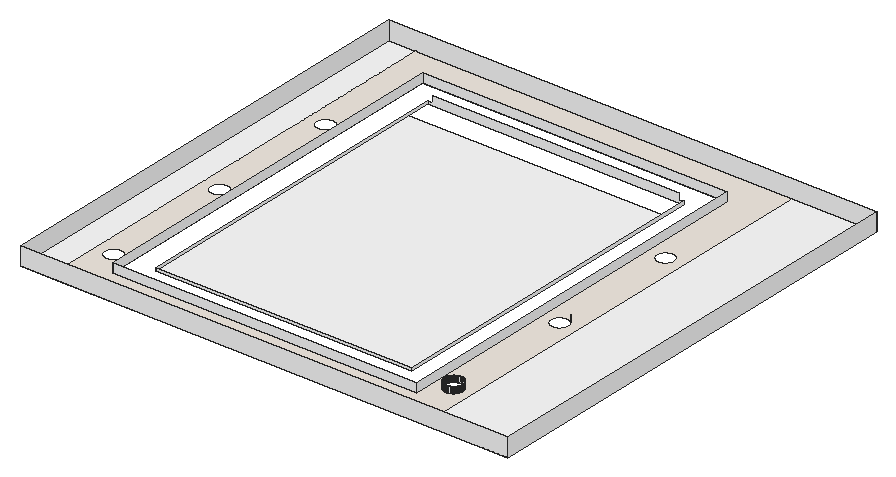
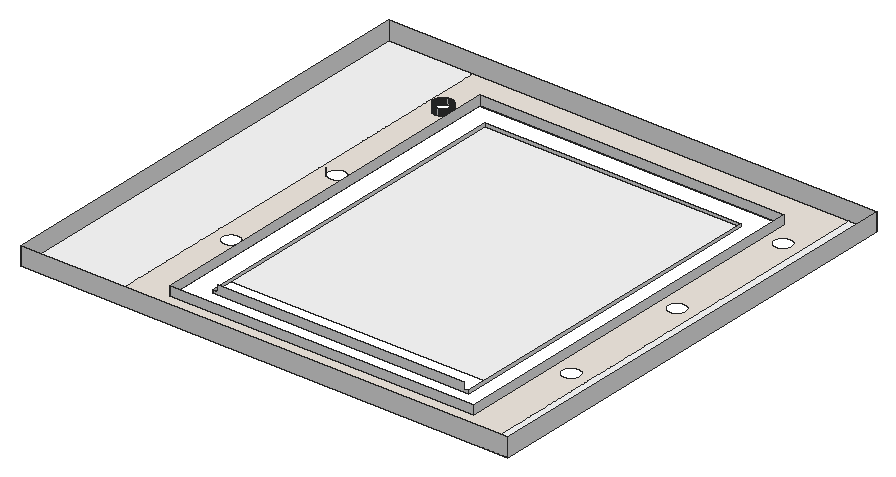
# SketchUp Ruby script. Lengths in inches.
U = 1.inch
M = Sketchup.active_model
def pt(a) = Geom::Point3d.new(a.map { |v| v * U })
def face(e, loops, mat)
  f = e.add_face(loops[0].map { |a| pt(a) })
  loops[1..].each { |l| e.add_face(l.map { |a| pt(a) }).erase! }
  f.material = f.back_material = mat if mat
  f
end
# faces: each face lists its corners as indices into pts; further lists are holes
def faces(e, pts, list, mat = nil) = list.each { |f| face(e, (f[0].is_a?(Array) ? f : [f]).map { |l| l.map { |i| pts[i] } }, mat) }
# xy, xz, yz: faces in a plane at the given z, y or x. An outline is a flat list of corners, or four numbers for a rectangle; further outlines are holes
def ring(l) = l.size == 4 ? [[l[0], l[1]], [l[2], l[1]], [l[2], l[3]], [l[0], l[3]]] : l.each_slice(2).to_a
def flat(e, list, mat, &to3) = list.each { |f| face(e, (f[0].is_a?(Array) ? f : [f]).map { |l| ring(l).map { |u, v| to3.(u, v) } }, mat) }
def xy(e, z, list, mat = nil) = flat(e, list, mat) { |x, y| [x, y, z] }
def xz(e, y, list, mat = nil) = flat(e, list, mat) { |x, z| [x, y, z] }
def yz(e, x, list, mat = nil) = flat(e, list, mat) { |y, z| [x, y, z] }
def lines(e, pts, list) = list.each { |a, b| e.add_line(pt(pts[a]), pt(pts[b])) }
# prism: a flat outline (further loops are holes) pulled along v
def prism(e, loops, v, mat = nil)
  f = face(e, loops, mat); d = Geom::Vector3d.new(v.map { |x| x * U })
  f.pushpull(f.normal.samedirection?(d) ? d.length : -d.length)
end
def box(e, o, s, mat = nil) = prism(e, [[o, [o[0] + s[0], o[1], o[2]], [o[0] + s[0], o[1] + s[1], o[2]], [o[0], o[1] + s[1], o[2]]]], [0, 0, s[2]], mat)
def at(x, y, z, deg = 0) = Geom::Transformation.translation(pt([x, y, z])) * Geom::Transformation.rotation(ORIGIN, Z_AXIS, deg.degrees)
def axes(o, x, y, z) = Geom::Transformation.new([*x, 0, *y, 0, *z, 0, *pt(o).to_a, 1])
def part(name) = M.definitions.add(name)
# library, detail: a bought-in or finely detailed component or shape, given as its bounding box
def library(name, o, s) = part(name).tap { |d| box(d.entities, o, s) }
def detail(e, o, s) = box(e.add_group.entities, o, s)
def put(e, d, t, mat = nil) = e.add_instance(d, t).tap { |i| i.material = mat if mat }
def group(e, t, mat = nil) = e.add_group.tap { |g| g.transformation = t; g.material = mat if mat }.entities
root = M.entities
M.materials.add("[Color M00]").color = [255, 255, 255]
M.materials.add("[Formica Laminate Light]").color = [242, 234, 226]
xy(root,120,[[0,0,9,153],[134,0,162,153],[29,20,114,125]],"[Color M00]")
xy(root,120,[[[9,0,134,153],[21,12,122,141],[14.87,105,15.0625,105,15.25,105.01,15.4375,105.03,15.62,105.07,15.81,105.11,15.98,105.17,16.16,105.23,16.33,105.3125,16.5,105.4,16.66,105.5,16.8125,105.61,16.96,105.73,17.1,105.86,17.23,105.99,17.35,106.14,17.57,106.44,17.66,106.61,17.74,106.78,17.8125,106.95,17.87,107.13,17.92,107.3125,17.96,107.5,17.98,107.68,18,107.87,18,108.0625,17.99,108.25,17.97,108.4375,17.93,108.62,17.89,108.81,17.83,108.98,17.77,109.16,17.6875,109.33,17.6,109.5,17.5,109.66,17.39,109.8125,17.27,109.96,17.14,110.1,17.01,110.23,16.86,110.35,16.56,110.57,16.39,110.66,16.22,110.74,16.05,110.8125,15.87,110.87,15.6875,110.92,15.5,110.96,15.32,110.98,15.13,111,14.9375,111,14.75,110.99,14.5625,110.97,14.38,110.93,14.19,110.89,14.02,110.83,13.84,110.77,13.67,110.6875,13.5,110.6,13.34,110.5,13.1875,110.39,13.04,110.27,12.9,110.14,12.77,110.01,12.65,109.86,12.43,109.56,12.34,109.39,12.26,109.22,12.1875,109.05,12.13,108.87,12.08,108.6875,12.04,108.5,12.02,108.32,12,108.13,12,107.9375,12.01,107.75,12.03,107.5625,12.07,107.38,12.11,107.19,12.17,107.02,12.23,106.84,12.3125,106.67,12.4,106.5,12.5,106.34,12.61,106.1875,12.73,106.04,12.86,105.9,12.99,105.77,13.14,105.65,13.44,105.43,13.61,105.34,13.78,105.26,13.95,105.1875,14.13,105.13,14.3125,105.08,14.5,105.04,14.68,105.02],[14.87,17,15.0625,17,15.25,17.01,15.4375,17.03,15.62,17.07,15.81,17.11,15.98,17.17,16.16,17.23,16.33,17.3125,16.5,17.4,16.66,17.5,16.8125,17.61,16.96,17.73,17.1,17.86,17.23,17.99,17.35,18.14,17.57,18.44,17.66,18.61,17.74,18.78,17.8125,18.95,17.87,19.13,17.92,19.3125,17.96,19.5,17.98,19.68,18,19.87,18,20.0625,17.99,20.25,17.97,20.4375,17.93,20.62,17.89,20.81,17.83,20.98,17.77,21.16,17.6875,21.33,17.6,21.5,17.5,21.66,17.39,21.8125,17.27,21.96,17.14,22.1,17.01,22.23,16.86,22.35,16.56,22.57,16.39,22.66,16.22,22.74,16.05,22.8125,15.87,22.87,15.6875,22.92,15.5,22.96,15.32,22.98,15.13,23,14.9375,23,14.75,22.99,14.5625,22.97,14.38,22.93,14.19,22.89,14.02,22.83,13.84,22.77,13.67,22.6875,13.5,22.6,13.34,22.5,13.1875,22.39,13.04,22.27,12.9,22.14,12.77,22.01,12.65,21.86,12.43,21.56,12.34,21.39,12.26,21.22,12.1875,21.05,12.13,20.87,12.08,20.6875,12.04,20.5,12.02,20.32,12,20.13,12,19.9375,12.01,19.75,12.03,19.5625,12.07,19.38,12.11,19.19,12.17,19.02,12.23,18.84,12.3125,18.67,12.4,18.5,12.5,18.34,12.61,18.1875,12.73,18.04,12.86,17.9,12.99,17.77,13.14,17.65,13.44,17.43,13.61,17.34,13.78,17.26,13.95,17.1875,14.13,17.13,14.3125,17.08,14.5,17.04,14.68,17.02],[14.87,61,15.0625,61,15.25,61.01,15.4375,61.03,15.62,61.07,15.81,61.11,15.98,61.17,16.16,61.23,16.33,61.3125,16.5,61.4,16.66,61.5,16.8125,61.61,16.96,61.73,17.1,61.86,17.23,61.99,17.35,62.14,17.57,62.44,17.66,62.61,17.74,62.78,17.8125,62.95,17.87,63.13,17.92,63.3125,17.96,63.5,17.98,63.68,18,63.87,18,64.0625,17.99,64.25,17.97,64.4375,17.93,64.62,17.89,64.81,17.83,64.98,17.77,65.16,17.6875,65.33,17.6,65.5,17.5,65.66,17.39,65.8125,17.27,65.96,17.14,66.1,17.01,66.23,16.86,66.35,16.56,66.57,16.39,66.66,16.22,66.74,16.05,66.8125,15.87,66.87,15.6875,66.92,15.5,66.96,15.32,66.98,15.13,67,14.9375,67,14.75,66.99,14.5625,66.97,14.38,66.93,14.19,66.89,14.02,66.83,13.84,66.77,13.67,66.6875,13.5,66.6,13.34,66.5,13.1875,66.39,13.04,66.27,12.9,66.14,12.77,66.01,12.65,65.86,12.43,65.56,12.34,65.39,12.26,65.22,12.1875,65.05,12.13,64.87,12.08,64.6875,12.04,64.5,12.02,64.32,12,64.13,12,63.9375,12.01,63.75,12.03,63.5625,12.07,63.38,12.11,63.19,12.17,63.02,12.23,62.84,12.3125,62.67,12.4,62.5,12.5,62.34,12.61,62.1875,12.73,62.04,12.86,61.9,12.99,61.77,13.14,61.65,13.44,61.43,13.61,61.34,13.78,61.26,13.95,61.1875,14.13,61.13,14.3125,61.08,14.5,61.04,14.68,61.02],[127.87,61,128.0625,61,128.25,61.01,128.4375,61.03,128.62,61.07,128.81,61.11,128.98,61.17,129.16,61.23,129.33,61.3125,129.5,61.4,129.66,61.5,129.8125,61.61,129.96,61.73,130.1,61.86,130.23,61.99,130.35,62.14,130.57,62.44,130.66,62.61,130.74,62.78,130.8125,62.95,130.87,63.13,130.92,63.3125,130.96,63.5,130.98,63.68,131,63.87,131,64.0625,130.99,64.25,130.97,64.4375,130.93,64.62,130.89,64.81,130.83,64.98,130.77,65.16,130.6875,65.33,130.6,65.5,130.5,65.66,130.39,65.8125,130.27,65.96,130.14,66.1,130.01,66.23,129.86,66.35,129.56,66.57,129.39,66.66,129.22,66.74,129.05,66.8125,128.87,66.87,128.6875,66.92,128.5,66.96,128.32,66.98,128.13,67,127.9375,67,127.75,66.99,127.5625,66.97,127.38,66.93,127.19,66.89,127.02,66.83,126.84,66.77,126.67,66.6875,126.5,66.6,126.34,66.5,126.1875,66.39,126.04,66.27,125.9,66.14,125.77,66.01,125.65,65.86,125.43,65.56,125.34,65.39,125.26,65.22,125.1875,65.05,125.13,64.87,125.08,64.6875,125.04,64.5,125.02,64.32,125,64.13,125,63.9375,125.01,63.75,125.03,63.5625,125.07,63.38,125.11,63.19,125.17,63.02,125.23,62.84,125.3125,62.67,125.4,62.5,125.5,62.34,125.61,62.1875,125.73,62.04,125.86,61.9,125.99,61.77,126.14,61.65,126.44,61.43,126.61,61.34,126.78,61.26,126.95,61.1875,127.13,61.13,127.3125,61.08,127.5,61.04,127.68,61.02],[127.87,17,128.0625,17,128.25,17.01,128.4375,17.03,128.62,17.07,128.81,17.11,128.98,17.17,129.16,17.23,129.33,17.3125,129.5,17.4,129.66,17.5,129.8125,17.61,129.96,17.73,130.1,17.86,130.23,17.99,130.35,18.14,130.57,18.44,130.66,18.61,130.74,18.78,130.8125,18.95,130.87,19.13,130.92,19.3125,130.96,19.5,130.98,19.68,131,19.87,131,20.0625,130.99,20.25,130.97,20.4375,130.93,20.62,130.89,20.81,130.83,20.98,130.77,21.16,130.6875,21.33,130.6,21.5,130.5,21.66,130.39,21.8125,130.27,21.96,130.14,22.1,130.01,22.23,129.86,22.35,129.56,22.57,129.39,22.66,129.22,22.74,129.05,22.8125,128.87,22.87,128.6875,22.92,128.5,22.96,128.32,22.98,128.13,23,127.9375,23,127.75,22.99,127.5625,22.97,127.38,22.93,127.19,22.89,127.02,22.83,126.84,22.77,126.67,22.6875,126.5,22.6,126.34,22.5,126.1875,22.39,126.04,22.27,125.9,22.14,125.77,22.01,125.65,21.86,125.43,21.56,125.34,21.39,125.26,21.22,125.1875,21.05,125.13,20.87,125.08,20.6875,125.04,20.5,125.02,20.32,125,20.13,125,19.9375,125.01,19.75,125.03,19.5625,125.07,19.38,125.11,19.19,125.17,19.02,125.23,18.84,125.3125,18.67,125.4,18.5,125.5,18.34,125.61,18.1875,125.73,18.04,125.86,17.9,125.99,17.77,126.14,17.65,126.44,17.43,126.61,17.34,126.78,17.26,126.95,17.1875,127.13,17.13,127.3125,17.08,127.5,17.04,127.68,17.02],[127.87,105,128.0625,105,128.25,105.01,128.4375,105.03,128.62,105.07,128.81,105.11,128.98,105.17,129.16,105.23,129.33,105.3125,129.5,105.4,129.66,105.5,129.8125,105.61,129.96,105.73,130.1,105.86,130.23,105.99,130.35,106.14,130.57,106.44,130.66,106.61,130.74,106.78,130.8125,106.95,130.87,107.13,130.92,107.3125,130.96,107.5,130.98,107.68,131,107.87,131,108.0625,130.99,108.25,130.97,108.4375,130.93,108.62,130.89,108.81,130.83,108.98,130.77,109.16,130.6875,109.33,130.6,109.5,130.5,109.66,130.39,109.8125,130.27,109.96,130.14,110.1,130.01,110.23,129.86,110.35,129.56,110.57,129.39,110.66,129.22,110.74,129.05,110.8125,128.87,110.87,128.6875,110.92,128.5,110.96,128.32,110.98,128.13,111,127.9375,111,127.75,110.99,127.5625,110.97,127.38,110.93,127.19,110.89,127.02,110.83,126.84,110.77,126.67,110.6875,126.5,110.6,126.34,110.5,126.1875,110.39,126.04,110.27,125.9,110.14,125.77,110.01,125.65,109.86,125.43,109.56,125.34,109.39,125.26,109.22,125.1875,109.05,125.13,108.87,125.08,108.6875,125.04,108.5,125.02,108.32,125,108.13,125,107.9375,125.01,107.75,125.03,107.5625,125.07,107.38,125.11,107.19,125.17,107.02,125.23,106.84,125.3125,106.67,125.4,106.5,125.5,106.34,125.61,106.1875,125.73,106.04,125.86,105.9,125.99,105.77,126.14,105.65,126.44,105.43,126.61,105.34,126.78,105.26,126.95,105.1875,127.13,105.13,127.3125,105.08,127.5,105.04,127.68,105.02]]],"[Formica Laminate Light]")
xz(root,0,[[0,120,162,126]],"[Color M00]")
xz(root,12,[[21,120,122,123]],"[Color M00]")
xz(root,17,[[127.87,120,128.0625,122]],"[Color M00]")
xz(root,20,[[29,120,114,121]],"[Color M00]")
xz(root,23,[[127.9375,120,128.13,122]],"[Color M00]")
xz(root,133,[[29,120,29,121,30.5,121,30.5,123,112.5,123,112.5,121,114,121,114,120]],"[Color M00]")
xz(root,141,[[21,120,122,123]],"[Color M00]")
xz(root,153,[[0,120,162,126]],"[Color M00]")
yz(root,0,[[0,120,153,126]],"[Color M00]")
yz(root,21,[[12,120,141,123]],"[Color M00]")
yz(root,29,[[20,120,133,121]],"[Color M00]")
yz(root,114,[[20,120,133,121]],"[Color M00]")
yz(root,122,[[12,120,141,123]],"[Color M00]")
yz(root,125,[[19.9375,120,20.13,122]],"[Color M00]")
yz(root,131,[[19.87,120,20.0625,122]],"[Color M00]")
yz(root,162,[[0,120,153,126]],"[Color M00]")
p = [[127.5,17.04,120],[127.3125,17.08,120],[127.3125,17.08,122],[127.5,17.04,122],[127.68,17.02,120],[127.68,17.02,122],
  [127.87,17,120],[127.87,17,122],[128.25,17.01,120],[128.0625,17,120],[128.0625,17,122],[128.25,17.01,122],
  [128.4375,17.03,120],[128.4375,17.03,122],[128.62,17.07,120],[128.62,17.07,122],[127.13,17.13,120],[126.95,17.1875,120],
  [126.95,17.1875,122],[127.13,17.13,122],[128.81,17.11,120],[128.81,17.11,122],[128.98,17.17,120],[128.98,17.17,122],
  [126.78,17.26,120],[126.78,17.26,122],[129.16,17.23,120],[129.16,17.23,122],[129.33,17.3125,120],[129.33,17.3125,122],
  [126.61,17.34,120],[126.44,17.43,120],[126.44,17.43,122],[126.61,17.34,122],[129.5,17.4,120],[129.5,17.4,122],
  [126.29,17.54,120],[126.29,17.54,122],[129.66,17.5,120],[129.66,17.5,122],[126.14,17.65,120],[126.14,17.65,122],
  [129.8125,17.61,120],[129.8125,17.61,122],[125.99,17.77,120],[125.99,17.77,122],[129.96,17.73,120],[129.96,17.73,122],
  [130.1,17.86,120],[130.1,17.86,122],[125.86,17.9,120],[125.86,17.9,122],[125.73,18.04,120],[125.73,18.04,122],
  [130.23,17.99,120],[130.23,17.99,122],[125.61,18.1875,120],[125.61,18.1875,122],[130.35,18.14,120],[130.35,18.14,122],
  [130.46,18.29,120],[130.46,18.29,122],[125.5,18.34,120],[125.5,18.34,122],[125.4,18.5,120],[125.4,18.5,122],
  [130.57,18.44,120],[130.57,18.44,122],[130.66,18.61,120],[130.66,18.61,122],[125.3125,18.67,120],[125.3125,18.67,122],
  [130.74,18.78,120],[130.74,18.78,122],[125.23,18.84,120],[125.23,18.84,122],[125.17,19.02,120],[125.17,19.02,122],
  [130.8125,18.95,120],[130.8125,18.95,122],[125.11,19.19,120],[125.11,19.19,122],[130.87,19.13,120],[130.87,19.13,122],
  [130.92,19.3125,120],[130.92,19.3125,122],[125.07,19.38,120],[125.07,19.38,122],[130.96,19.5,120],[130.96,19.5,122],
  [125.03,19.5625,120],[125.03,19.5625,122],[130.98,19.68,120],[130.98,19.68,122],[125.01,19.75,120],[125.01,19.75,122],
  [131,19.87,120],[131,19.87,122],[125,19.9375,120],[125,19.9375,122],[125,20.13,120],[125.02,20.32,120],
  [125.02,20.32,122],[125,20.13,122],[130.99,20.25,120],[131,20.0625,120],[131,20.0625,122],[130.99,20.25,122],
  [130.97,20.4375,120],[130.97,20.4375,122],[125.04,20.5,120],[125.04,20.5,122],[130.93,20.62,120],[130.93,20.62,122],
  [125.08,20.6875,120],[125.08,20.6875,122],[130.89,20.81,120],[130.89,20.81,122],[125.13,20.87,120],[125.13,20.87,122],
  [130.83,20.98,120],[130.83,20.98,122],[125.1875,21.05,120],[125.1875,21.05,122],[125.26,21.22,120],[125.26,21.22,122],
  [130.77,21.16,120],[130.77,21.16,122],[125.34,21.39,120],[125.34,21.39,122],[130.6875,21.33,120],[130.6875,21.33,122],
  [130.6,21.5,120],[130.6,21.5,122],[125.43,21.56,120],[125.43,21.56,122],[130.5,21.66,120],[130.5,21.66,122],
  [125.54,21.71,120],[125.54,21.71,122],[125.65,21.86,120],[125.65,21.86,122],[130.39,21.8125,120],[130.39,21.8125,122],
  [130.27,21.96,120],[130.27,21.96,122],[125.77,22.01,120],[125.77,22.01,122],[125.9,22.14,120],[125.9,22.14,122],
  [130.14,22.1,120],[130.14,22.1,122],[126.04,22.27,120],[126.04,22.27,122],[130.01,22.23,120],[130.01,22.23,122],
  [129.86,22.35,120],[129.86,22.35,122],[126.1875,22.39,120],[126.1875,22.39,122],[126.34,22.5,120],[126.34,22.5,122],
  [129.71,22.46,120],[129.71,22.46,122],[126.5,22.6,120],[126.5,22.6,122],[129.56,22.57,120],[129.56,22.57,122],
  [126.67,22.6875,120],[126.67,22.6875,122],[129.39,22.66,120],[129.39,22.66,122],[126.84,22.77,120],[126.84,22.77,122],
  [129.05,22.8125,120],[129.22,22.74,120],[129.22,22.74,122],[129.05,22.8125,122],[127.02,22.83,120],[127.02,22.83,122],
  [127.19,22.89,120],[127.19,22.89,122],[128.87,22.87,120],[128.87,22.87,122],[127.38,22.93,120],[127.38,22.93,122],
  [127.5625,22.97,120],[127.5625,22.97,122],[128.5,22.96,120],[128.6875,22.92,120],[128.6875,22.92,122],[128.5,22.96,122],
  [127.75,22.99,120],[127.75,22.99,122],[127.9375,23,120],[127.9375,23,122],[128.13,23,120],[128.32,22.98,120],
  [128.32,22.98,122],[128.13,23,122],[130.39,65.8125,120],[130.5,65.66,120],[130.5,65.66,122],[130.39,65.8125,122],
  [130.27,65.96,120],[130.27,65.96,122],[130.14,66.1,120],[130.14,66.1,122],[130.01,66.23,120],[130.01,66.23,122],
  [129.86,66.35,120],[129.86,66.35,122]]
faces(root,p,[[0,1,2,3],[4,0,3,5],[6,4,5,7],[8,9,10,11],[12,8,11,13],[14,12,13,15],[16,17,18,19],[1,16,19,2],
  [20,14,15,21],[22,20,21,23],[17,24,25,18],[26,22,23,27],[28,26,27,29],[30,31,32,33],[24,30,33,25],[34,28,29,35],
  [31,36,37,32],[38,34,35,39],[36,40,41,37],[42,38,39,43],[40,44,45,41],[46,42,43,47],[48,46,47,49],[44,50,51,45],
  [50,52,53,51],[54,48,49,55],[52,56,57,53],[58,54,55,59],[60,58,59,61],[56,62,63,57],[62,64,65,63],[66,60,61,67],
  [68,66,67,69],[64,70,71,65],[72,68,69,73],[70,74,75,71],[74,76,77,75],[78,72,73,79],[76,80,81,77],[82,78,79,83],
  [84,82,83,85],[80,86,87,81],[88,84,85,89],[86,90,91,87],[92,88,89,93],[90,94,95,91],[96,92,93,97],[94,98,99,95],
  [100,101,102,103],[104,105,106,107],[108,104,107,109],[101,110,111,102],[112,108,109,113],[110,114,115,111],[116,112,113,117],[114,118,119,115],
  [120,116,117,121],[118,122,123,119],[122,124,125,123],[126,120,121,127],[124,128,129,125],[130,126,127,131],[132,130,131,133],[128,134,135,129],
  [136,132,133,137],[134,138,139,135],[138,140,141,139],[142,136,137,143],[144,142,143,145],[140,146,147,141],[146,148,149,147],[150,144,145,151],
  [148,152,153,149],[154,150,151,155],[156,154,155,157],[152,158,159,153],[158,160,161,159],[162,156,157,163],[160,164,165,161],[166,162,163,167],
  [164,168,169,165],[170,166,167,171],[168,172,173,169],[174,175,176,177],[175,170,171,176],[172,178,179,173],[178,180,181,179],[182,174,177,183],
  [180,184,185,181],[184,186,187,185],[188,189,190,191],[189,182,183,190],[186,192,193,187],[192,194,195,193],[196,197,198,199],[197,188,191,198],
  [200,201,202,203],[204,200,203,205],[206,204,205,207],[208,206,207,209],[210,208,209,211]],"[Color M00]")
